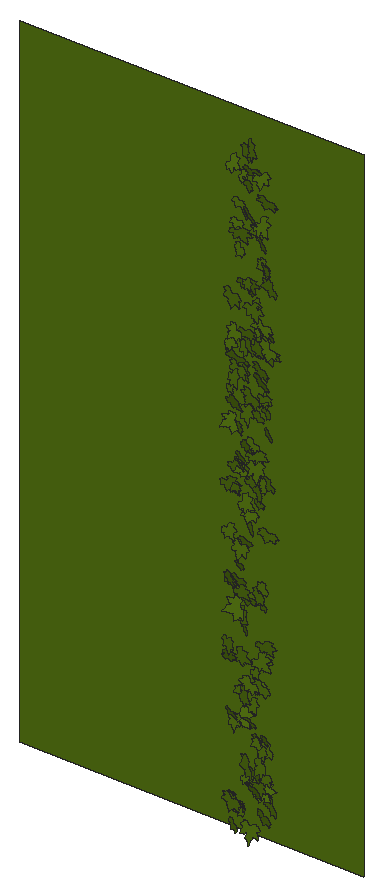
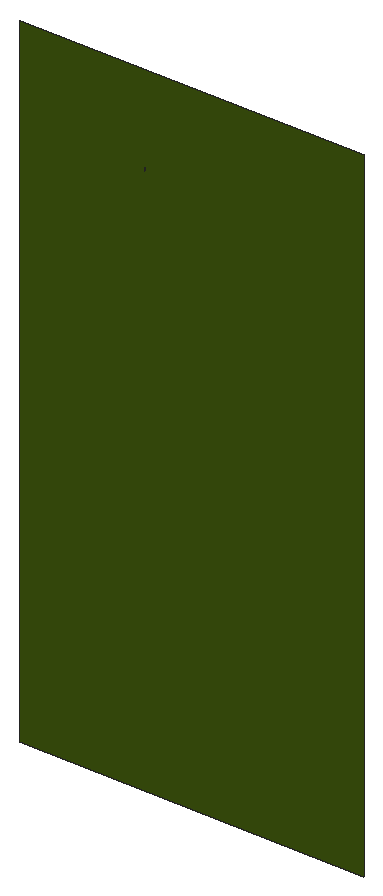
# SketchUp Ruby script. Lengths in inches.
U = 1.inch
M = Sketchup.active_model
def pt(a) = Geom::Point3d.new(a.map { |v| v * U })
def face(e, loops, mat)
  f = e.add_face(loops[0].map { |a| pt(a) })
  loops[1..].each { |l| e.add_face(l.map { |a| pt(a) }).erase! }
  f.material = f.back_material = mat if mat
  f
end
# faces: each face lists its corners as indices into pts; further lists are holes
def faces(e, pts, list, mat = nil) = list.each { |f| face(e, (f[0].is_a?(Array) ? f : [f]).map { |l| l.map { |i| pts[i] } }, mat) }
# xy, xz, yz: faces in a plane at the given z, y or x. An outline is a flat list of corners, or four numbers for a rectangle; further outlines are holes
def ring(l) = l.size == 4 ? [[l[0], l[1]], [l[2], l[1]], [l[2], l[3]], [l[0], l[3]]] : l.each_slice(2).to_a
def flat(e, list, mat, &to3) = list.each { |f| face(e, (f[0].is_a?(Array) ? f : [f]).map { |l| ring(l).map { |u, v| to3.(u, v) } }, mat) }
def xy(e, z, list, mat = nil) = flat(e, list, mat) { |x, y| [x, y, z] }
def xz(e, y, list, mat = nil) = flat(e, list, mat) { |x, z| [x, y, z] }
def yz(e, x, list, mat = nil) = flat(e, list, mat) { |y, z| [x, y, z] }
def lines(e, pts, list) = list.each { |a, b| e.add_line(pt(pts[a]), pt(pts[b])) }
# prism: a flat outline (further loops are holes) pulled along v
def prism(e, loops, v, mat = nil)
  f = face(e, loops, mat); d = Geom::Vector3d.new(v.map { |x| x * U })
  f.pushpull(f.normal.samedirection?(d) ? d.length : -d.length)
end
def box(e, o, s, mat = nil) = prism(e, [[o, [o[0] + s[0], o[1], o[2]], [o[0] + s[0], o[1] + s[1], o[2]], [o[0], o[1] + s[1], o[2]]]], [0, 0, s[2]], mat)
def at(x, y, z, deg = 0) = Geom::Transformation.translation(pt([x, y, z])) * Geom::Transformation.rotation(ORIGIN, Z_AXIS, deg.degrees)
def axes(o, x, y, z) = Geom::Transformation.new([*x, 0, *y, 0, *z, 0, *pt(o).to_a, 1])
def part(name) = M.definitions.add(name)
# library, detail: a bought-in or finely detailed component or shape, given as its bounding box
def library(name, o, s) = part(name).tap { |d| box(d.entities, o, s) }
def detail(e, o, s) = box(e.add_group.entities, o, s)
def put(e, d, t, mat = nil) = e.add_instance(d, t).tap { |i| i.material = mat if mat }
def group(e, t, mat = nil) = e.add_group.tap { |g| g.transformation = t; g.material = mat if mat }.entities
root = M.entities
M.materials.add("[Vegetation Blur 03]").color = [83, 114, 18]
c1 = part("ivy")
xy(c1.entities,0,[[0.782,0,0.786,0,0.787,0.005,0.789,0.009,0.821,0.072,0.875,0.147,1.001,0.272,1.073,0.331,1.137,0.363,1.178,0.379,1.223,0.384,1.272,0.383,1.311,0.374,1.36,0.355,1.399,0.334,1.491,0.285,1.541,0.244,1.583,0.199,1.617,0.15,1.64,0.128,1.662,0.115,1.717,0.105,1.745,0.093,1.784,0.054,1.819,0.057,1.854,0.064,1.882,0.075,1.896,0.074,1.91,0.071,1.937,0.063,1.964,0.053,1.99,0.038,2.016,0.015,2.034,0.002,2.04,0,2.038,0.003,2.036,0.007,2.033,0.038,2.036,0.068,2.045,0.1,2.055,0.116,2.064,0.123,2.077,0.129,2.088,0.129,2.106,0.132,2.118,0.13,2.179,0.132,2.207,0.133,2.225,0.133,2.242,0.138,2.22,0.162,2.207,0.186,2.206,0.213,2.212,0.236,2.228,0.262,2.247,0.274,2.298,0.283,2.355,0.294,2.37,0.296,2.376,0.295,2.377,0.3,2.377,0.303,2.385,0.329,2.411,0.37,2.426,0.392,2.449,0.407,2.511,0.426,2.561,0.444,2.619,0.466,2.589,0.469,2.561,0.476,2.501,0.5,2.449,0.516,2.424,0.523,2.401,0.535,2.377,0.556,2.372,0.568,2.36,0.575,2.268,0.586,2.225,0.592,2.207,0.599,2.194,0.61,2.143,0.65,2.13,0.664,2.122,0.682,2.123,0.7,2.13,0.719,2.148,0.75,2.17,0.781,2.195,0.807,2.221,0.828,2.284,0.874,2.291,0.88,2.288,0.887,2.276,0.9,2.267,0.916,2.265,0.933,2.273,0.967,2.292,1.002,2.313,1.03,2.334,1.054,2.348,1.067,2.358,1.074,2.363,1.076,2.362,1.081,2.35,1.094,2.347,1.11,2.35,1.143,2.359,1.18,2.385,1.254,2.415,1.324,2.448,1.393,2.45,1.4,2.446,1.398,2.44,1.394,2.427,1.383,2.402,1.36,2.376,1.339,2.345,1.324,2.305,1.309,2.282,1.303,2.273,1.306,2.245,1.294,2.212,1.287,2.187,1.291,2.163,1.301,2.142,1.316,2.134,1.327,2.124,1.325,2.09,1.292,2.053,1.259,2.014,1.234,1.973,1.215,1.954,1.21,1.931,1.208,1.909,1.212,1.893,1.22,1.879,1.233,1.872,1.248,1.867,1.281,1.864,1.319,1.821,1.258,1.773,1.197,1.726,1.141,1.698,1.121,1.679,1.116,1.666,1.117,1.647,1.122,1.632,1.129,1.62,1.141,1.617,1.154,1.617,1.219,1.621,1.254,1.623,1.268,1.623,1.281,1.618,1.314,1.606,1.346,1.603,1.375,1.607,1.403,1.603,1.467,1.599,1.499,1.605,1.525,1.614,1.552,1.629,1.577,1.635,1.589,1.629,1.587,1.618,1.582,1.596,1.566,1.581,1.556,1.568,1.552,1.557,1.55,1.545,1.553,1.531,1.562,1.522,1.572,1.504,1.591,1.486,1.611,1.474,1.631,1.457,1.666,1.455,1.684,1.457,1.698,1.452,1.715,1.444,1.728,1.424,1.754,1.419,1.772,1.423,1.786,1.434,1.819,1.444,1.848,1.446,1.855,1.44,1.861,1.43,1.867,1.386,1.904,1.349,1.948,1.326,1.973,1.31,1.995,1.288,2.048,1.284,2.153,1.287,2.254,1.284,2.255,1.282,2.253,1.278,2.247,1.274,2.237,1.266,2.216,1.226,2.125,1.208,2.076,1.184,2.033,1.155,1.984,1.135,1.942,1.111,1.899,1.083,1.861,1.053,1.85,1.059,1.83,1.061,1.809,1.056,1.79,1.049,1.767,1.04,1.749,1.018,1.733,0.994,1.726,0.942,1.734,0.95,1.6875,0.944,1.645,0.932,1.608,0.911,1.585,0.881,1.58,0.854,1.582,0.828,1.588,0.785,1.618,0.773,1.625,0.775,1.614,0.779,1.598,0.796,1.502,0.818,1.402,0.861,1.283,0.882,1.224,0.894,1.174,0.892,1.148,0.886,1.123,0.881,1.107,0.872,1.099,0.849,1.094,0.818,1.092,0.789,1.098,0.762,1.107,0.753,1.113,0.721,1.139,0.698,1.163,0.678,1.194,0.665,1.224,0.628,1.28,0.612,1.312,0.606,1.327,0.606,1.314,0.599,1.282,0.594,1.267,0.581,1.256,0.544,1.245,0.512,1.244,0.473,1.249,0.444,1.256,0.382,1.288,0.339,1.306,0.324,1.316,0.317,1.324,0.309,1.326,0.27,1.314,0.227,1.313,0.185,1.3125,0.152,1.317,0.122,1.328,0.092,1.345,0.073,1.353,0.079,1.338,0.092,1.308,0.117,1.249,0.13,1.215,0.139,1.164,0.147,1.148,0.157,1.136,0.163,1.122,0.174,1.086,0.177,1.067,0.182,1.054,0.186,1.043,0.191,1.038,0.211,1.028,0.237,1.005,0.25,0.974,0.253,0.96,0.25,0.944,0.242,0.914,0.243,0.906,0.249,0.902,0.26,0.894,0.289,0.88,0.307,0.873,0.322,0.862,0.364,0.799,0.403,0.738,0.431,0.709,0.439,0.691,0.441,0.678,0.4375,0.66,0.428,0.645,0.394,0.623,0.303,0.594,0.255,0.581,0.214,0.577,0.179,0.573,0.173,0.568,0.175,0.561,0.167,0.55,0.141,0.523,0.113,0.503,0.077,0.49,0.045,0.486,0.026,0.485,0.019,0.486,0.011,0.483,0,0.471,0.014,0.467,0.044,0.455,0.058,0.447,0.07,0.438,0.097,0.411,0.125,0.394,0.158,0.377,0.174,0.366,0.182,0.359,0.185,0.361,0.242,0.331,0.253,0.316,0.258,0.303,0.262,0.283,0.274,0.278,0.308,0.274,0.341,0.252,0.366,0.226,0.366,0.222,0.37,0.22,0.38,0.221,0.395,0.221,0.425,0.216,0.45,0.207,0.465,0.192,0.473,0.178,0.484,0.15,0.489,0.116,0.483,0.089,0.468,0.058,0.45,0.035,0.435,0.018,0.429,0.011,0.434,0.012,0.438,0.014,0.469,0.019,0.542,0.016,0.581,0.015,0.612,0.027,0.68,0.055,0.696,0.057,0.712,0.052,0.73,0.045,0.741,0.036,0.766,0.014]])
xz(root,174.5,[[62.28,53,86.74,99]],"[Vegetation Blur 03]")
put(root,c1,axes([77.39,173.7,69.06],[0.25004,-0.05522,0.19659],[0.24228,0.07618,-0.20189],[0.00655,-0.71038,-0.03693]),"[Vegetation Blur 03]")
put(root,c1,axes([77.89,173.7,55.81],[0.43018,0.03461,-0.33433],[-0.40999,0.03807,-0.35076],[-0.00059,-1.2218,-0.0204]),"[Vegetation Blur 03]")
put(root,c1,axes([77.32,173.7,64.03],[0.13975,-0.17275,0.35559],[0.44281,0.11446,-0.10717],[0.0284,-0.9346,-0.07885]),"[Vegetation Blur 03]")
put(root,c1,axes([77.14,173.7,72.2],[0.35229,-0.00554,0.29733],[0.36145,-0.12544,-0.28562],[-0.04568,-1.0353,0.03302]),"[Vegetation Blur 03]")
put(root,c1,axes([78.07,173.7,80.11],[0.3559,-0.06669,-0.38571],[-0.47242,-0.14005,-0.28653],[0.03508,-1.20938,0.05445]),"[Vegetation Blur 03]")
put(root,c1,axes([77.41,173.7,55.72],[0.62299,-0.15418,-0.12642],[-0.15294,0.05244,-0.51207],[-0.07884,-1.31998,-0.00558]),"[Vegetation Blur 03]")
put(root,c1,axes([77.38,173.7,83.97],[0.08788,0.15958,0.41108],[0.50211,-0.20702,-0.05886],[-0.08717,-1.03158,0.0754]),"[Vegetation Blur 03]")
put(root,c1,axes([76.98,173.7,75.21],[0.49372,-0.08066,0.3359],[0.41334,0.06825,-0.4021],[-0.00879,-1.32093,-0.04129]),"[Vegetation Blur 03]")
put(root,c1,axes([77.875,173.7,54.14],[0.34936,-0.1754,-0.17065],[-0.20005,0.12722,-0.29335],[-0.10473,-0.82812,-0.00892]),"[Vegetation Blur 03]")
put(root,c1,axes([77.7,173.7,75.82],[0.46927,-0.11869,-0.14311],[-0.17217,0.07416,-0.3857],[-0.06659,-1.02821,-0.0113]),"[Vegetation Blur 03]")
put(root,c1,axes([77.56,173.7,81.45],[0.20111,-0.0492,0.23305],[0.27447,-0.17313,-0.16352],[-0.08231,-0.69755,0.02415]),"[Vegetation Blur 03]")
put(root,c1,axes([77.29,173.7,65.51],[0.49387,-0.24848,0.14861],[0.17062,-0.13992,-0.41447],[-0.13648,-1.07408,0.01961]),"[Vegetation Blur 03]")
put(root,c1,axes([77.61,173.7,83.9375],[0.61818,0.02753,-0.20694],[-0.25253,0.20999,-0.49806],[-0.0265,-1.35881,-0.08116]),"[Vegetation Blur 03]")
put(root,c1,axes([77.48,173.7,95.34],[0.1221,0.15901,0.36769],[0.45566,-0.11863,-0.09271],[-0.03634,-0.95319,0.07288]),"[Vegetation Blur 03]")
put(root,c1,axes([77.77,173.7,55.77],[0.53938,-0.11783,-0.24861],[-0.28048,0.34993,-0.43141],[-0.13192,-1.22575,-0.09926]),"[Vegetation Blur 03]")
put(root,c1,axes([77.49,173.7,61.0625],[0.49941,-0.26714,0.04177],[0.06827,0.12648,-0.4165],[-0.1217,-1.02529,-0.06226]),"[Vegetation Blur 03]")
put(root,c1,axes([78.68,173.7,93.38],[0.10747,0.09693,-0.42949],[-0.50045,0.37307,-0.07017],[-0.16944,-1.0404,-0.06517]),"[Vegetation Blur 03]")
put(root,c1,axes([77.47,173.7,87.95],[0.66254,-0.24066,-0.04091],[-0.05165,-0.00895,-0.54898],[-0.11628,-1.36725,0.01079]),"[Vegetation Blur 03]")
put(root,c1,axes([77.4,173.7,69.45],[0.34584,-0.27967,0.31588],[0.38688,-0.124,-0.2994],[-0.13639,-1.06088,-0.04828]),"[Vegetation Blur 03]")
put(root,c1,axes([78.08,173.7,85.8],[0.41213,-0.1677,-0.21359],[-0.27008,-0.08234,-0.33694],[-0.04682,-1.00125,0.06348]),"[Vegetation Blur 03]")
put(root,c1,axes([78.57,173.7,68.5],[0.32603,-0.13943,-0.47145],[-0.58131,-0.12239,-0.26207],[0.01889,-1.35947,0.07195]),"[Vegetation Blur 03]")
put(root,c1,axes([78.01,173.7,92.4],[0.32282,0.01218,-0.05233],[-0.06347,-0.05325,-0.26277],[0.01083,-0.67519,0.01978]),"[Vegetation Blur 03]")
put(root,c1,axes([77.6,173.7,76.54],[0.35919,-0.07581,0.24051],[0.29623,0.02355,-0.29351],[-0.02119,-0.9558,-0.02631]),"[Vegetation Blur 03]")
put(root,c1,axes([78.18,173.7,93.8],[0.32239,-0.01176,-0.10948],[-0.13423,-0.01041,-0.2631],[-0.00333,-0.71849,0.00561]),"[Vegetation Blur 03]")
put(root,c1,axes([78.7,173.7,55.01],[0.06839,0.01536,-0.24268],[-0.29667,-0.04173,-0.0561],[0.02144,-0.62648,-0.00221]),"[Vegetation Blur 03]")
put(root,c1,axes([78.6,173.7,62.71],[0.15181,-0.00524,-0.23084],[-0.28286,-0.00517,-0.12389],[0.00101,-0.66057,0.0028]),"[Vegetation Blur 03]")
put(root,c1,axes([77.49,173.7,80.62],[0.38193,-0.25872,0.35613],[0.44798,0.02235,-0.31745],[-0.07443,-1.19311,-0.08317]),"[Vegetation Blur 03]")
put(root,c1,axes([78.93,173.7,66.9],[0.06026,0.01776,-0.40154],[-0.46093,0.35917,-0.04358],[-0.17229,-0.95467,-0.02387]),"[Vegetation Blur 03]")
put(root,c1,axes([78.36,173.7,77.6],[0.28037,-0.06157,-0.15463],[-0.18018,0.15229,-0.22714],[-0.06579,-0.67947,-0.0369]),"[Vegetation Blur 03]")
put(root,c1,axes([77.66,173.7,82.13],[0.31073,-0.06738,0.37222],[0.4328,-0.32267,-0.24985],[-0.14749,-1.08882,0.05101]),"[Vegetation Blur 03]")
put(root,c1,axes([77.96,173.7,69.7],[0.47998,-0.11829,-0.01678],[-0.01365,0.11877,-0.39191],[-0.0595,-0.98146,-0.0454]),"[Vegetation Blur 03]")
put(root,c1,axes([77.79,173.7,60.68],[0.45593,-0.14871,0.15697],[0.17169,-0.25336,-0.36992],[-0.11285,-0.98625,0.07136]),"[Vegetation Blur 03]")
put(root,c1,axes([78.1875,173.7,70.55],[0.3065,-0.10801,0.00878],[0.01921,0.10156,-0.25024],[-0.05001,-0.62289,-0.04232]),"[Vegetation Blur 03]")
put(root,c1,axes([77.91,173.7,83.42],[0.63233,-0.20373,-0.05495],[-0.06893,-0.01048,-0.5222],[-0.0979,-1.30853,0.01274]),"[Vegetation Blur 03]")
put(root,c1,axes([77.64,173.7,91.53],[0.56255,-0.01811,0.20546],[0.25121,0.13405,-0.45628],[0.01862,-1.26114,-0.05145]),"[Vegetation Blur 03]")
put(root,c1,axes([78.77,173.7,76.98],[0.19807,-0.04882,-0.25327],[-0.31096,-0.06252,-0.16009],[0.01294,-0.755,0.02963]),"[Vegetation Blur 03]")
put(root,c1,axes([78.14,173.7,77.22],[0.42582,-0.25778,-0.01572],[0.00049,0.14225,-0.35818],[-0.12674,-0.86554,-0.05419]),"[Vegetation Blur 03]")
put(root,c1,axes([78.65,173.7,72.24],[0.26692,0.10027,-0.19485],[-0.24358,0.09015,-0.21495],[0.00657,-0.73139,-0.05321]),"[Vegetation Blur 03]")
put(root,c1,axes([78.39,173.7,91.04],[0.38208,-0.19358,-0.10183],[-0.13229,-0.03969,-0.31874],[-0.08317,-0.82615,0.03917]),"[Vegetation Blur 03]")
put(root,c1,axes([77.7,173.7,60.34],[0.39393,0.1891,0.39235],[0.48905,-0.10099,-0.3194],[0.01969,-1.27498,0.08349]),"[Vegetation Blur 03]")
put(root,c1,axes([78.1,173.7,79.4375],[0.37901,-0.24998,0.16924],[0.20826,-0.05609,-0.32368],[-0.11995,-0.88726,-0.02722]),"[Vegetation Blur 03]")
put(root,c1,axes([78.13,173.7,82.7],[0.23197,-0.0436,0.29061],[0.3566,0.00644,-0.18945],[-0.00894,-0.8745,-0.01588]),"[Vegetation Blur 03]")
put(root,c1,axes([79.08,173.7,58.44],[0.28462,-0.17247,-0.45638],[-0.54186,0.28495,-0.24203],[-0.16158,-1.25936,0.00774]),"[Vegetation Blur 03]")
put(root,c1,axes([78.1,173.7,71.98],[0.58607,-0.17658,0.01299],[0.00501,-0.15402,-0.47969],[-0.08713,-1.19658,0.05983]),"[Vegetation Blur 03]")
put(root,c1,axes([77.94,173.7,68.58],[0.39343,-0.07208,0.30532],[0.37571,0.06003,-0.32024],[-0.0052,-1.11557,-0.03696]),"[Vegetation Blur 03]")
put(root,c1,axes([78.43,173.7,94.95],[0.0888,0.09674,0.25308],[0.31076,-0.1168,-0.0656],[-0.0424,-0.6534,0.0492]),"[Vegetation Blur 03]")
put(root,c1,axes([78.86,173.7,84.92],[0.29115,-0.21346,-0.2217],[-0.27097,0.0878,-0.25032],[-0.10549,-0.81469,0.03111]),"[Vegetation Blur 03]")
put(root,c1,axes([79.38,173.7,77.1],[0.14596,0.116,-0.44941],[-0.55223,-0.05004,-0.12149],[0.03805,-1.17121,-0.03932]),"[Vegetation Blur 03]")
put(root,c1,axes([78.11,173.7,64.21],[0.18573,-0.07263,0.44986],[0.55141,-0.04477,-0.15278],[-0.03192,-1.19609,-0.0216]),"[Vegetation Blur 03]")
put(root,c1,axes([78.61,173.7,68.51],[0.38415,0.08832,-0.09325],[-0.11924,0.10565,-0.31143],[0.02608,-0.81794,-0.0503]),"[Vegetation Blur 03]")
put(root,c1,axes([78.87,173.7,93.38],[0.42548,-0.09437,-0.33716],[-0.38139,0.39508,-0.33797],[-0.16527,-1.15464,-0.08808]),"[Vegetation Blur 03]")
put(root,c1,axes([78.9375,173.7,97.45],[0.35368,-0.15187,-0.29343],[-0.34945,0.17479,-0.29479],[-0.11221,-1.02299,-0.00681]),"[Vegetation Blur 03]")
put(root,c1,axes([79.05,173.7,60.8],[0.21856,0.08137,-0.22546],[-0.27868,0.10188,-0.17416],[-0.01478,-0.71768,-0.05028]),"[Vegetation Blur 03]")
put(root,c1,axes([78.53,173.7,56.72],[0.17985,0.03398,0.21034],[0.25744,-0.07475,-0.14472],[-0.02044,-0.64238,0.02797]),"[Vegetation Blur 03]")
put(root,c1,axes([79.03,173.7,85.11],[0.38374,-0.03816,-0.34105],[-0.41282,0.15382,-0.31209],[-0.06752,-1.15732,-0.03024]),"[Vegetation Blur 03]")
put(root,c1,axes([79.4,173.7,73.25],[0.07886,-0.02245,-0.3122],[-0.36365,0.24601,-0.06396],[-0.11923,-0.76517,-0.0114]),"[Vegetation Blur 03]")
put(root,c1,axes([78.33,173.7,73.98],[0.16307,0.08475,0.41488],[0.5096,-0.07153,-0.13111],[-0.02064,-1.09626,0.04063]),"[Vegetation Blur 03]")
put(root,c1,axes([78.96,173.7,63.56],[0.42678,-0.01115,-0.26433],[-0.32354,-0.0687,-0.34749],[0.01587,-1.10035,0.02437]),"[Vegetation Blur 03]")
put(root,c1,axes([78.4,173.7,66.98],[0.16191,-0.03187,0.41572],[0.48687,-0.31523,-0.1301],[-0.15054,-1.05373,0.02635]),"[Vegetation Blur 03]")
put(root,c1,axes([78.35,173.7,85.48],[0.51847,-0.08238,0.09913],[0.12469,0.09368,-0.42215],[-0.02842,-1.09178,-0.0437]),"[Vegetation Blur 03]")
put(root,c1,axes([78.16,173.7,88.53],[0.5764,-0.04158,0.19028],[0.23362,0.17732,-0.46527],[0.01378,-1.26714,-0.07135]),"[Vegetation Blur 03]")
put(root,c1,axes([78.36,173.7,82.95],[0.39018,-0.19806,0.28181],[0.33951,-0.13277,-0.32778],[-0.115,-1.06391,-0.01155]),"[Vegetation Blur 03]")
put(root,c1,axes([78.5,173.7,61.8125],[0.12637,-0.06641,0.44261],[0.52763,-0.25805,-0.10643],[-0.12947,-1.11645,-0.00173]),"[Vegetation Blur 03]")
put(root,c1,axes([79.01,173.7,88.41],[0.29856,-0.10941,-0.11062],[-0.12269,0.1536,-0.24445],[-0.0784,-0.65702,-0.03873]),"[Vegetation Blur 03]")
put(root,c1,axes([78.96,173.7,82.02],[0.54012,-0.12372,-0.29412],[-0.3556,0.12595,-0.44329],[-0.0839,-1.33021,-0.01462]),"[Vegetation Blur 03]")
put(root,c1,axes([78.8,173.7,74.15],[0.44019,0.01869,-0.05575],[-0.06711,-0.08998,-0.3577],[0.01564,-0.91223,0.03414]),"[Vegetation Blur 03]")
put(root,c1,axes([78.57,173.7,78.07],[0.25746,-0.20708,0.31713],[0.39391,-0.05224,-0.21837],[-0.07715,-0.95777,-0.05666]),"[Vegetation Blur 03]")
put(root,c1,axes([78.7,173.7,95.22],[0.42985,-0.21428,0.06487],[0.08397,0.02008,-0.36019],[-0.10055,-0.89931,-0.0235]),"[Vegetation Blur 03]")
put(root,c1,axes([78.72,173.7,88.5],[0.26598,-0.07146,0.22657],[0.27016,-0.13937,-0.21816],[-0.07275,-0.7788,0.01825]),"[Vegetation Blur 03]")
put(root,c1,axes([79.25,173.7,78.82],[0.32974,-0.02071,-0.22461],[-0.27537,-0.01528,-0.26905],[-0.00296,-0.88368,0.00992]),"[Vegetation Blur 03]")
put(root,c1,axes([78.51,173.7,80.55],[0.51632,-0.17161,0.26126],[0.29868,-0.283,-0.42241],[-0.14219,-1.21766,0.06135]),"[Vegetation Blur 03]")
put(root,c1,axes([78.65,173.7,54.21],[0.65317,-0.15035,0.08957],[0.09783,-0.2124,-0.5313],[-0.08838,-1.34629,0.07382]),"[Vegetation Blur 03]")
put(root,c1,axes([79.83,173.7,80.67],[0.16409,0.0678,-0.30247],[-0.37206,0.03564,-0.13319],[-0.00256,-0.83328,-0.0303]),"[Vegetation Blur 03]")
put(root,c1,axes([78.82,173.7,75.74],[0.26787,-0.06927,0.33281],[0.40897,0.07748,-0.21671],[0.01312,-1.00101,-0.0398]),"[Vegetation Blur 03]")
put(root,c1,axes([78.68,173.7,95.96],[0.62307,-0.149,0.09151],[0.12235,0.19755,-0.50432],[-0.05332,-1.28769,-0.08796]),"[Vegetation Blur 03]")
put(root,c1,axes([79.74,173.7,59.95],[0.28434,-0.07307,-0.35446],[-0.41994,0.239,-0.23213],[-0.11635,-1.04116,-0.02841]),"[Vegetation Blur 03]")
put(root,c1,axes([79.84,173.7,92.49],[0.19509,-0.01615,-0.32843],[-0.40182,0.04546,-0.15934],[-0.0233,-0.91916,-0.00211]),"[Vegetation Blur 03]")
put(root,c1,axes([78.89,173.7,56.75],[0.57489,-0.26657,0.03866],[0.06843,0.18847,-0.47339],[-0.11976,-1.17196,-0.08492]),"[Vegetation Blur 03]")
put(root,c1,axes([79.79,173.7,76.49],[0.3874,-0.28987,-0.42046],[-0.49062,0.32448,-0.33628],[-0.21109,-1.28615,0.00992]),"[Vegetation Blur 03]")
put(root,c1,axes([78.95,173.7,61.6875],[0.31135,-0.03304,0.2876],[0.34314,-0.19604,-0.25097],[-0.08184,-0.94759,0.04189]),"[Vegetation Blur 03]")
put(root,c1,axes([79.82,173.7,59.82],[0.20749,-0.03484,-0.23563],[-0.28917,-0.01288,-0.16931],[-0.00479,-0.73151,0.0142]),"[Vegetation Blur 03]")
put(root,c1,axes([79.04,173.7,96.75],[0.0835,-0.00667,0.46395],[0.54474,-0.33722,-0.06606],[-0.16259,-1.13325,0.01693]),"[Vegetation Blur 03]")
put(root,c1,axes([78.71,173.7,87.15],[0.58643,-0.10608,0.2337],[0.28408,-0.0778,-0.48036],[-0.06289,-1.34069,0.00938]),"[Vegetation Blur 03]")
put(root,c1,axes([78.83,173.7,77.65],[0.54429,0.0275,0.19656],[0.23996,0.06284,-0.44397],[0.02457,-1.22318,-0.01839]),"[Vegetation Blur 03]")
put(root,c1,axes([79.27,173.7,63.82],[0.22624,-0.03067,0.2044],[0.24637,-0.10398,-0.18409],[-0.04741,-0.6867,0.01875]),"[Vegetation Blur 03]")
put(root,c1,axes([80.18,173.7,68.83],[0.12874,0.00958,-0.35889],[-0.43298,0.16781,-0.10275],[-0.07698,-0.92784,-0.02229]),"[Vegetation Blur 03]")
put(root,c1,axes([79.68,173.7,83.04],[0.44147,-0.0788,-0.2903],[-0.33877,0.28169,-0.35517],[-0.11502,-1.13213,-0.06817]),"[Vegetation Blur 03]")
put(root,c1,axes([79.87,173.7,57.77],[0.29889,-0.0519,-0.2268],[-0.27904,-0.05258,-0.24304],[-0.001,-0.83818,0.02929]),"[Vegetation Blur 03]")
put(root,c1,axes([79.45,173.7,87.43],[0.18943,-0.02258,0.18927],[0.22327,-0.15119,-0.15168],[-0.06367,-0.59736,0.03124]),"[Vegetation Blur 03]")
put(root,c1,axes([79.11,173.7,57.71],[0.48095,-0.24511,0.14889],[0.18901,0.01686,-0.4023],[-0.10837,-1.05836,-0.04089]),"[Vegetation Blur 03]")
put(root,c1,axes([79.6,173.7,74.97],[0.32248,-0.05987,-0.04087],[-0.04757,0.05862,-0.26354],[-0.03303,-0.669,-0.01944]),"[Vegetation Blur 03]")
put(root,c1,axes([79.66,173.7,86.23],[0.34481,-0.20074,-0.10306],[-0.10927,0.15385,-0.29065],[-0.11628,-0.7398,-0.03248]),"[Vegetation Blur 03]")
put(root,c1,axes([79.7,173.7,63.59],[0.47072,-0.03676,-0.23219],[-0.28418,0.02801,-0.38445],[-0.02233,-1.13149,-0.00197]),"[Vegetation Blur 03]")
put(root,c1,axes([80.27,173.7,69.86],[0.16539,-0.02327,-0.29289],[-0.35869,0.02592,-0.13523],[-0.01618,-0.81273,0.00407]),"[Vegetation Blur 03]")
put(root,c1,axes([79.53,173.7,83.81],[0.56634,-0.19077,-0.13861],[-0.15859,0.16167,-0.4666],[-0.11086,-1.2059,-0.04063]),"[Vegetation Blur 03]")
put(root,c1,axes([79.56,173.7,62.78],[0.17104,0.07406,0.23051],[0.28468,-0.03259,-0.13906],[0.00499,-0.6787,0.03183]),"[Vegetation Blur 03]")
put(root,c1,axes([79.55,173.7,69.41],[0.49502,-0.2424,-0.04719],[-0.06027,-0.00753,-0.41504],[-0.11656,-1.02555,0.0142]),"[Vegetation Blur 03]")
put(root,c1,axes([79.07,173.7,77.15],[0.58365,-0.1286,0.23072],[0.26562,-0.28309,-0.47237],[-0.11521,-1.30414,0.07979]),"[Vegetation Blur 03]")
put(root,c1,axes([79.67,173.7,86.5625],[0.53942,-0.03341,-0.15907],[-0.19556,-0.07489,-0.43924],[-0.00287,-1.17788,0.03244]),"[Vegetation Blur 03]")
put(root,c1,axes([79.26,173.7,84.5],[0.30631,-0.15054,0.36025],[0.43855,-0.11732,-0.25607],[-0.08874,-1.09937,-0.022]),"[Vegetation Blur 03]")
put(root,c1,axes([80.41,173.7,76.4375],[0.12105,-0.13191,-0.28197],[-0.3442,0.10689,-0.10629],[-0.07075,-0.74572,0.03464]),"[Vegetation Blur 03]")
put(root,c1,axes([79.3125,173.7,56.97],[0.52242,-0.17809,0.13316],[0.16214,-0.04009,-0.43214],[-0.08844,-1.12553,-0.00568]),"[Vegetation Blur 03]")
put(root,c1,axes([80.25,173.7,90.55],[0.26106,-0.06742,-0.29363],[-0.35973,0.03582,-0.21432],[-0.03335,-0.91402,0.01326]),"[Vegetation Blur 03]")
put(root,c1,axes([79.875,173.7,91.82],[0.38591,-0.21569,-0.14541],[-0.15737,0.19687,-0.32414],[-0.13402,-0.85224,-0.03808]),"[Vegetation Blur 03]")
put(root,c1,axes([80.58,173.7,76.625],[0.1471,0.09742,-0.39347],[-0.48397,0.0748,-0.1176],[-0.02114,-1.03455,-0.04555]),"[Vegetation Blur 03]")
put(root,c1,axes([79.23,173.7,64.35],[0.3582,0.03063,0.42978],[0.52659,-0.05959,-0.29166],[-0.01559,-1.30923,0.02333]),"[Vegetation Blur 03]")
put(root,c1,axes([79.58,173.7,64.62],[0.36162,0.06548,0.17991],[0.22033,0.0215,-0.29621],[0.03262,-0.87124,0.00621]),"[Vegetation Blur 03]")
put(root,c1,axes([80.37,173.7,85.49],[0.37878,0.01189,-0.41383],[-0.50562,-0.09055,-0.30867],[0.03871,-1.29927,0.01773]),"[Vegetation Blur 03]")
put(root,c1,axes([79.89,173.7,94.52],[0.51764,0.02568,-0.18283],[-0.22378,0.14257,-0.41887],[-0.01616,-1.15189,-0.05592]),"[Vegetation Blur 03]")
put(root,c1,axes([79.82,173.7,55.34],[0.50401,-0.18357,-0.11952],[-0.1351,0.15116,-0.41597],[-0.10561,-1.06941,-0.03828]),"[Vegetation Blur 03]")
put(root,c1,axes([79.53,173.7,95.9375],[0.54024,-0.08088,0.09089],[0.10321,-0.19815,-0.43637],[-0.05739,-1.11765,0.07079]),"[Vegetation Blur 03]")
put(root,c1,axes([79.42,173.7,56.1],[0.37101,0.18964,0.31894],[0.39968,-0.06988,-0.30314],[0.03834,-1.10666,0.0738]),"[Vegetation Blur 03]")
put(root,c1,axes([80.75,173.7,89.29],[0.18125,0.04011,-0.45454],[-0.55361,0.15105,-0.14494],[-0.06386,-1.19573,-0.03356]),"[Vegetation Blur 03]")
put(root,c1,axes([80.35,173.7,81.625],[0.34504,-0.21965,-0.31495],[-0.37042,0.22285,-0.29474],[-0.152,-1.04167,0.00335]),"[Vegetation Blur 03]")
put(root,c1,axes([80.59,173.7,59.85],[0.21313,-0.07118,-0.35531],[-0.43534,0.04461,-0.17534],[-0.03471,-0.99647,0.01753]),"[Vegetation Blur 03]")
put(root,c1,axes([79.4,173.7,92.22],[0.34036,0.06769,0.40355],[0.48921,-0.24292,-0.26842],[-0.07909,-1.21115,0.07639]),"[Vegetation Blur 03]")
put(root,c1,axes([79.9,173.7,57.97],[0.51001,-0.14732,-0.08686],[-0.10909,-0.02593,-0.41973],[-0.06746,-1.07179,0.02209]),"[Vegetation Blur 03]")
put(root,c1,axes([80.4,173.7,86.11],[0.28115,-0.04858,-0.24392],[-0.28246,0.2397,-0.22437],[-0.10049,-0.80964,-0.05179]),"[Vegetation Blur 03]")
put(root,c1,axes([80,173.7,73.31],[0.48743,0.04761,-0.1367],[-0.16843,0.04371,-0.39762],[0.01495,-1.05971,-0.02254]),"[Vegetation Blur 03]")
put(root,c1,axes([80.43,173.7,79.74],[0.24639,-0.0769,-0.23479],[-0.27054,0.21951,-0.20041],[-0.10474,-0.7479,-0.03468]),"[Vegetation Blur 03]")
put(root,c1,axes([79.78,173.7,59.01],[0.30019,-0.07683,0.21744],[0.25164,-0.21034,-0.24309],[-0.09515,-0.7987,0.0431]),"[Vegetation Blur 03]")
put(root,c1,axes([80.72,173.7,56.45],[0.27997,-0.09905,-0.45822],[-0.54252,0.30141,-0.23104],[-0.15235,-1.25535,-0.01932]),"[Vegetation Blur 03]")
put(root,c1,axes([79.97,173.7,59.01],[0.55698,-0.45746,-0.14027],[-0.2006,-0.09744,-0.48055],[-0.19678,-1.19551,0.09284]),"[Vegetation Blur 03]")
put(root,c1,axes([79.58,173.7,84.5],[0.59787,0.07047,0.08314],[0.09735,0.14687,-0.48587],[0.04553,-1.23935,-0.05285]),"[Vegetation Blur 03]")
put(root,c1,axes([80.0625,173.7,81.21],[0.05918,0.07636,0.27369],[0.32495,-0.20144,-0.03796],[-0.0908,-0.67116,0.04253]),"[Vegetation Blur 03]")
put(root,c1,axes([79.53,173.7,65.73],[0.50143,-0.04661,0.23263],[0.28578,0.12116,-0.40648],[0.00953,-1.18071,-0.05089]),"[Vegetation Blur 03]")
put(root,c1,axes([79.77,173.7,81.69],[0.45211,-0.0957,0.11404],[0.13937,-0.02195,-0.37092],[-0.04759,-0.97354,-0.00285]),"[Vegetation Blur 03]")
put(root,c1,axes([79.99,173.7,59.97],[0.28812,-0.17967,0.12477],[0.15963,0.01216,-0.24278],[-0.07425,-0.67108,-0.0378]),"[Vegetation Blur 03]")
put(root,c1,axes([80,173.7,90.25],[0.44121,-0.22953,-0.01023],[-0.00431,0.06987,-0.3705],[-0.11216,-0.9056,-0.026]),"[Vegetation Blur 03]")
